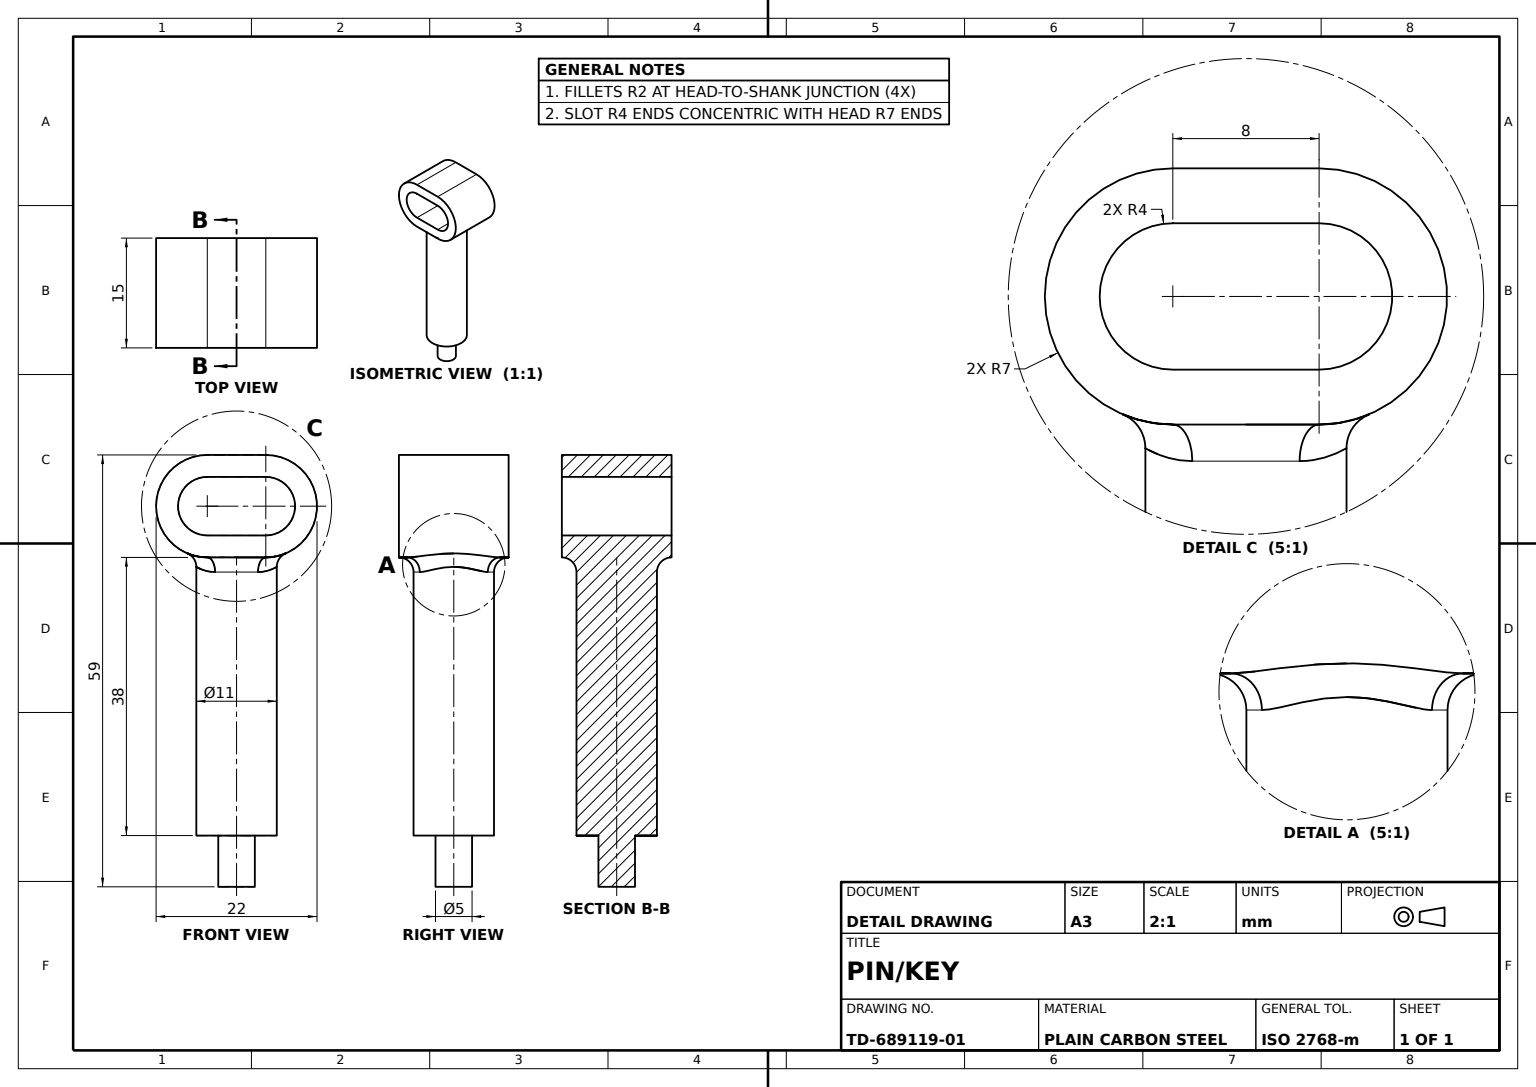
ISO-10303-21;
HEADER;
FILE_DESCRIPTION((''),'2;1');
FILE_NAME('','',(''),(''),'','','');
FILE_SCHEMA(('AUTOMOTIVE_DESIGN'));
ENDSEC;
DATA;
#1=APPLICATION_CONTEXT('');
#2=PRODUCT_CONTEXT('',#1,'mechanical');
#3=PRODUCT('','','',(#2));
#4=PRODUCT_DEFINITION_FORMATION('','',#3);
#5=PRODUCT_DEFINITION_CONTEXT('',#1,'design');
#6=PRODUCT_DEFINITION('','',#4,#5);
#7=PRODUCT_DEFINITION_SHAPE('','',#6);
#8=(LENGTH_UNIT()NAMED_UNIT(*)SI_UNIT(.MILLI.,.METRE.));
#9=(NAMED_UNIT(*)PLANE_ANGLE_UNIT()SI_UNIT($,.RADIAN.));
#10=(NAMED_UNIT(*)SI_UNIT($,.STERADIAN.)SOLID_ANGLE_UNIT());
#11=UNCERTAINTY_MEASURE_WITH_UNIT(LENGTH_MEASURE(1.E-05),#8,'distance_accuracy_value','');
#12=(GEOMETRIC_REPRESENTATION_CONTEXT(3)GLOBAL_UNCERTAINTY_ASSIGNED_CONTEXT((#11))GLOBAL_UNIT_ASSIGNED_CONTEXT((#8,#9,#10))REPRESENTATION_CONTEXT('',''));
#13=CARTESIAN_POINT('',(4.,-7.,-6.344289));
#14=VERTEX_POINT('',#13);
#15=CARTESIAN_POINT('',(4.,-7.,-7.5));
#16=VERTEX_POINT('',#15);
#17=CARTESIAN_POINT('',(4.,-7.,7.5));
#18=DIRECTION('',(0.,0.,-1.));
#19=VECTOR('',#18,1000.);
#20=LINE('',#17,#19);
#21=EDGE_CURVE('',#14,#16,#20,.T.);
#22=ORIENTED_EDGE('',*,*,#21,.F.);
#23=CARTESIAN_POINT('',(0.,-7.,-7.5));
#24=VERTEX_POINT('',#23);
#25=CARTESIAN_POINT('',(0.,-7.,0.));
#26=DIRECTION('',(0.,1.,0.));
#27=DIRECTION('',(-1.,0.,0.));
#28=AXIS2_PLACEMENT_3D('',#25,#26,#27);
#29=CIRCLE('',#28,7.5);
#30=EDGE_CURVE('',#14,#24,#29,.T.);
#31=ORIENTED_EDGE('',*,*,#30,.T.);
#32=CARTESIAN_POINT('',(-4.,-7.,-7.5));
#33=DIRECTION('',(1.,0.,0.));
#34=VECTOR('',#33,1000.);
#35=LINE('',#32,#34);
#36=EDGE_CURVE('',#24,#16,#35,.T.);
#37=ORIENTED_EDGE('',*,*,#36,.T.);
#38=EDGE_LOOP('',(#22,#31,#37));
#39=FACE_OUTER_BOUND('',#38,.T.);
#40=CARTESIAN_POINT('',(-4.,-7.,7.5));
#41=AXIS2_PLACEMENT_3D('',#40,#26,#27);
#42=PLANE('',#41);
#43=ADVANCED_FACE('',(#39),#42,.F.);
#44=CARTESIAN_POINT('',(4.,4.,7.5));
#45=VERTEX_POINT('',#44);
#46=CARTESIAN_POINT('',(-4.,4.,7.5));
#47=VERTEX_POINT('',#46);
#48=VECTOR('',#27,1000.);
#49=LINE('',#46,#48);
#50=EDGE_CURVE('',#45,#47,#49,.T.);
#51=ORIENTED_EDGE('',*,*,#50,.F.);
#52=CARTESIAN_POINT('',(4.,-4.,7.5));
#53=VERTEX_POINT('',#52);
#54=CARTESIAN_POINT('',(4.,0.,7.5));
#55=DIRECTION('',(0.,0.,1.));
#56=AXIS2_PLACEMENT_3D('',#54,#55,#33);
#57=CIRCLE('',#56,4.);
#58=EDGE_CURVE('',#53,#45,#57,.T.);
#59=ORIENTED_EDGE('',*,*,#58,.F.);
#60=CARTESIAN_POINT('',(-4.,-4.,7.5));
#61=VERTEX_POINT('',#60);
#62=LINE('',#60,#34);
#63=EDGE_CURVE('',#61,#53,#62,.T.);
#64=ORIENTED_EDGE('',*,*,#63,.F.);
#65=CARTESIAN_POINT('',(-8.,0.,7.5));
#66=VERTEX_POINT('',#65);
#67=CARTESIAN_POINT('',(-4.,0.,7.5));
#68=AXIS2_PLACEMENT_3D('',#67,#55,#33);
#69=CIRCLE('',#68,4.);
#70=EDGE_CURVE('',#66,#61,#69,.T.);
#71=ORIENTED_EDGE('',*,*,#70,.F.);
#72=EDGE_CURVE('',#47,#66,#69,.T.);
#73=ORIENTED_EDGE('',*,*,#72,.F.);
#74=EDGE_LOOP('',(#51,#59,#64,#71,#73));
#75=FACE_BOUND('',#74,.T.);
#76=VERTEX_POINT('',#40);
#77=CARTESIAN_POINT('',(0.,-7.,7.5));
#78=VERTEX_POINT('',#77);
#79=LINE('',#40,#34);
#80=EDGE_CURVE('',#76,#78,#79,.T.);
#81=ORIENTED_EDGE('',*,*,#80,.T.);
#82=VERTEX_POINT('',#17);
#83=EDGE_CURVE('',#78,#82,#79,.T.);
#84=ORIENTED_EDGE('',*,*,#83,.T.);
#85=CARTESIAN_POINT('',(4.,7.,7.5));
#86=VERTEX_POINT('',#85);
#87=CIRCLE('',#56,7.);
#88=EDGE_CURVE('',#82,#86,#87,.T.);
#89=ORIENTED_EDGE('',*,*,#88,.T.);
#90=CARTESIAN_POINT('',(-4.,7.,7.5));
#91=VERTEX_POINT('',#90);
#92=LINE('',#90,#48);
#93=EDGE_CURVE('',#86,#91,#92,.T.);
#94=ORIENTED_EDGE('',*,*,#93,.T.);
#95=CARTESIAN_POINT('',(-11.,0.,7.5));
#96=VERTEX_POINT('',#95);
#97=CIRCLE('',#68,7.);
#98=EDGE_CURVE('',#91,#96,#97,.T.);
#99=ORIENTED_EDGE('',*,*,#98,.T.);
#100=EDGE_CURVE('',#96,#76,#97,.T.);
#101=ORIENTED_EDGE('',*,*,#100,.T.);
#102=EDGE_LOOP('',(#81,#84,#89,#94,#99,#101));
#103=FACE_OUTER_BOUND('',#102,.T.);
#104=PLANE('',#68);
#105=ADVANCED_FACE('',(#75,#103),#104,.T.);
#106=ORIENTED_EDGE('',*,*,#63,.T.);
#107=CARTESIAN_POINT('',(4.,-4.,-7.5));
#108=VERTEX_POINT('',#107);
#109=LINE('',#52,#19);
#110=EDGE_CURVE('',#53,#108,#109,.T.);
#111=ORIENTED_EDGE('',*,*,#110,.T.);
#112=CARTESIAN_POINT('',(-4.,-4.,-7.5));
#113=VERTEX_POINT('',#112);
#114=LINE('',#112,#34);
#115=EDGE_CURVE('',#113,#108,#114,.T.);
#116=ORIENTED_EDGE('',*,*,#115,.F.);
#117=LINE('',#60,#19);
#118=EDGE_CURVE('',#61,#113,#117,.T.);
#119=ORIENTED_EDGE('',*,*,#118,.F.);
#120=EDGE_LOOP('',(#106,#111,#116,#119));
#121=FACE_OUTER_BOUND('',#120,.T.);
#122=AXIS2_PLACEMENT_3D('',#60,#26,#27);
#123=PLANE('',#122);
#124=ADVANCED_FACE('',(#121),#123,.T.);
#125=CARTESIAN_POINT('',(-2.933333,-9.,4.652478));
#126=VERTEX_POINT('',#125);
#127=CARTESIAN_POINT('',(-4.,-7.,6.344289));
#128=VERTEX_POINT('',#127);
#129=CARTESIAN_POINT('',(-4.,-9.,6.344289));
#130=DIRECTION('',(0.845905169,0.,0.533333333));
#131=DIRECTION('',(0.533333333,0.,-0.845905169));
#132=AXIS2_PLACEMENT_3D('',#129,#130,#131);
#133=CIRCLE('',#132,2.);
#134=EDGE_CURVE('',#126,#128,#133,.T.);
#135=ORIENTED_EDGE('',*,*,#134,.F.);
#136=CARTESIAN_POINT('',(2.933333,-9.,4.652478));
#137=VERTEX_POINT('',#136);
#138=CARTESIAN_POINT('',(0.,-9.,0.));
#139=DIRECTION('',(0.,-1.,0.));
#140=AXIS2_PLACEMENT_3D('',#138,#139,#27);
#141=CIRCLE('',#140,5.5);
#142=EDGE_CURVE('',#137,#126,#141,.T.);
#143=ORIENTED_EDGE('',*,*,#142,.F.);
#144=CARTESIAN_POINT('',(4.,-7.,6.344289));
#145=VERTEX_POINT('',#144);
#146=CARTESIAN_POINT('',(4.,-9.,6.344289));
#147=DIRECTION('',(-0.845905169,0.,0.533333333));
#148=DIRECTION('',(0.533333333,0.,0.845905169));
#149=AXIS2_PLACEMENT_3D('',#146,#147,#148);
#150=CIRCLE('',#149,2.);
#151=EDGE_CURVE('',#145,#137,#150,.T.);
#152=ORIENTED_EDGE('',*,*,#151,.F.);
#153=EDGE_CURVE('',#78,#145,#29,.T.);
#154=ORIENTED_EDGE('',*,*,#153,.F.);
#155=EDGE_CURVE('',#128,#78,#29,.T.);
#156=ORIENTED_EDGE('',*,*,#155,.F.);
#157=EDGE_LOOP('',(#135,#143,#152,#154,#156));
#158=FACE_OUTER_BOUND('',#157,.T.);
#159=AXIS2_PLACEMENT_3D('',#138,#26,#27);
#160=TOROIDAL_SURFACE('',#159,7.5,2.);
#161=ADVANCED_FACE('',(#158),#160,.F.);
#162=ORIENTED_EDGE('',*,*,#83,.F.);
#163=ORIENTED_EDGE('',*,*,#153,.T.);
#164=EDGE_CURVE('',#82,#145,#20,.T.);
#165=ORIENTED_EDGE('',*,*,#164,.F.);
#166=EDGE_LOOP('',(#162,#163,#165));
#167=FACE_OUTER_BOUND('',#166,.T.);
#168=ADVANCED_FACE('',(#167),#42,.F.);
#169=CARTESIAN_POINT('',(2.933333,-9.,-4.652478));
#170=VERTEX_POINT('',#169);
#171=CARTESIAN_POINT('',(5.5,-8.291562,0.));
#172=VERTEX_POINT('',#171);
#173=CARTESIAN_POINT('',(3.133043,-9.,-4.526564));
#174=CARTESIAN_POINT('',(3.324343,-8.987525,-4.387772));
#175=CARTESIAN_POINT('',(3.681966,-8.945264,-4.092301));
#176=CARTESIAN_POINT('',(3.84954,-8.915501,-3.934916));
#177=CARTESIAN_POINT('',(4.320562,-8.809648,-3.43407));
#178=CARTESIAN_POINT('',(4.59485,-8.715803,-3.05715));
#179=CARTESIAN_POINT('',(4.925989,-8.581444,-2.456998));
#180=CARTESIAN_POINT('',(5.023745,-8.53753,-2.25051));
#181=CARTESIAN_POINT('',(5.193968,-8.456487,-1.823596));
#182=CARTESIAN_POINT('',(5.266775,-8.419162,-1.601479));
#183=CARTESIAN_POINT('',(5.440779,-8.326918,-0.928725));
#184=CARTESIAN_POINT('',(5.5,-8.291562,-0.470006));
#185=B_SPLINE_CURVE_WITH_KNOTS('',3,(#169,#173,#174,#175,#176,#177,#178,#179,#180,#181,#182,#183,#184,#171),.UNSPECIFIED.,.F.,.F.,(4,2,2,2,2,2,4),(0.,0.000707891,0.001415783,0.002831566,0.003539457,0.004247348,0.005663131),.UNSPECIFIED.);
#186=EDGE_CURVE('',#170,#172,#185,.T.);
#187=ORIENTED_EDGE('',*,*,#186,.F.);
#188=CARTESIAN_POINT('',(4.,-9.,-6.344289));
#189=AXIS2_PLACEMENT_3D('',#188,#130,#131);
#190=CIRCLE('',#189,2.);
#191=EDGE_CURVE('',#14,#170,#190,.T.);
#192=ORIENTED_EDGE('',*,*,#191,.F.);
#193=CARTESIAN_POINT('',(4.468237,-7.,5.964722));
#194=CARTESIAN_POINT('',(4.865103,-6.955024,5.526591));
#195=CARTESIAN_POINT('',(5.378548,-6.865114,4.799618));
#196=CARTESIAN_POINT('',(5.535888,-6.830968,4.544603));
#197=CARTESIAN_POINT('',(5.817747,-6.761425,4.023897));
#198=CARTESIAN_POINT('',(5.943356,-6.725845,3.756806));
#199=CARTESIAN_POINT('',(6.278059,-6.623061,2.936233));
#200=CARTESIAN_POINT('',(6.445689,-6.55993,2.359248));
#201=CARTESIAN_POINT('',(6.666602,-6.473277,1.194519));
#202=CARTESIAN_POINT('',(6.722103,-6.449043,0.600743));
#203=CARTESIAN_POINT('',(6.722341,-6.448942,-0.596899));
#204=CARTESIAN_POINT('',(6.667486,-6.472915,-1.188495));
#205=CARTESIAN_POINT('',(6.501583,-6.538013,-2.065229));
#206=CARTESIAN_POINT('',(6.431801,-6.564616,-2.356752));
#207=CARTESIAN_POINT('',(6.264949,-6.624036,-2.92676));
#208=CARTESIAN_POINT('',(6.167832,-6.656884,-3.206115));
#209=CARTESIAN_POINT('',(5.833401,-6.759663,-4.027076));
#210=CARTESIAN_POINT('',(5.549791,-6.835022,-4.556645));
#211=CARTESIAN_POINT('',(5.039313,-6.92457,-5.280187));
#212=CARTESIAN_POINT('',(4.854699,-6.950556,-5.510504));
#213=CARTESIAN_POINT('',(4.452763,-6.988258,-5.947148));
#214=CARTESIAN_POINT('',(4.234007,-7.,-6.154596));
#215=B_SPLINE_CURVE_WITH_KNOTS('',3,(#144,#193,#194,#195,#196,#197,#198,#199,#200,#201,#202,#203,#204,#205,#206,#207,#208,#209,#210,#211,#212,#213,#214,#13),.UNSPECIFIED.,.F.,.F.,(4,2,2,2,2,2,2,2,2,2,2,4),(0.,0.001778288,0.002667432,0.003556577,0.005334865,0.007113153,0.008891442,0.009780586,0.01066973,0.012448018,0.013337162,0.014226307),.UNSPECIFIED.);
#216=EDGE_CURVE('',#145,#14,#215,.T.);
#217=ORIENTED_EDGE('',*,*,#216,.F.);
#218=ORIENTED_EDGE('',*,*,#151,.T.);
#219=CARTESIAN_POINT('',(5.5,-8.291562,0.23522));
#220=CARTESIAN_POINT('',(5.484785,-8.300403,0.469857));
#221=CARTESIAN_POINT('',(5.425872,-8.333622,0.929272));
#222=CARTESIAN_POINT('',(5.382182,-8.357987,1.15548));
#223=CARTESIAN_POINT('',(5.266772,-8.419159,1.601289));
#224=CARTESIAN_POINT('',(5.194588,-8.456191,1.822026));
#225=CARTESIAN_POINT('',(5.023221,-8.53778,2.251839));
#226=CARTESIAN_POINT('',(4.925051,-8.581848,2.458861));
#227=CARTESIAN_POINT('',(4.704312,-8.671365,2.858598));
#228=CARTESIAN_POINT('',(4.581742,-8.716834,3.051308));
#229=CARTESIAN_POINT('',(4.311141,-8.803745,3.422997));
#230=CARTESIAN_POINT('',(4.162384,-8.845267,3.602452));
#231=CARTESIAN_POINT('',(3.688497,-8.951547,4.105776));
#232=CARTESIAN_POINT('',(3.333153,-9.,4.400396));
#233=B_SPLINE_CURVE_WITH_KNOTS('',3,(#171,#219,#220,#221,#222,#223,#224,#225,#226,#227,#228,#229,#230,#231,#232,#136),.UNSPECIFIED.,.F.,.F.,(4,2,2,2,2,2,2,4),(0.005663131,0.006371677,0.007080223,0.007788769,0.008497314,0.00920586,0.009914406,0.011331498),.UNSPECIFIED.);
#234=EDGE_CURVE('',#172,#137,#233,.T.);
#235=ORIENTED_EDGE('',*,*,#234,.F.);
#236=EDGE_LOOP('',(#187,#192,#217,#218,#235));
#237=FACE_OUTER_BOUND('',#236,.T.);
#238=CARTESIAN_POINT('',(2.933333,-7.,4.652478));
#239=CARTESIAN_POINT('',(4.421288,-7.,6.002781));
#240=CARTESIAN_POINT('',(3.238913,-7.06306,4.459814));
#241=CARTESIAN_POINT('',(3.330464,-9.,4.402092));
#242=CARTESIAN_POINT('',(4.79799,-6.962674,5.602232));
#243=CARTESIAN_POINT('',(3.553947,-7.102304,4.223306));
#244=CARTESIAN_POINT('',(3.685723,-8.952009,4.108303));
#245=CARTESIAN_POINT('',(5.301296,-6.880082,4.915778));
#246=CARTESIAN_POINT('',(4.017096,-7.122128,3.768812));
#247=CARTESIAN_POINT('',(4.16027,-8.84582,3.604904));
#248=CARTESIAN_POINT('',(5.459491,-6.847756,4.670729));
#249=CARTESIAN_POINT('',(4.168117,-7.122554,3.602781));
#250=CARTESIAN_POINT('',(4.309425,-8.804258,3.425202));
#251=CARTESIAN_POINT('',(5.747471,-6.779987,4.162566));
#252=CARTESIAN_POINT('',(4.451479,-7.113522,3.246293));
#253=CARTESIAN_POINT('',(4.580949,-8.717126,3.052549));
#254=CARTESIAN_POINT('',(5.87798,-6.744494,3.898869));
#255=CARTESIAN_POINT('',(4.584829,-7.104349,3.055827));
#256=CARTESIAN_POINT('',(4.704001,-8.671493,2.85917));
#257=CARTESIAN_POINT('',(6.112868,-6.674639,3.351956));
#258=CARTESIAN_POINT('',(4.829413,-7.080665,2.6509));
#259=CARTESIAN_POINT('',(4.925466,-8.581678,2.458101));
#260=CARTESIAN_POINT('',(6.217247,-6.640264,3.068744));
#261=CARTESIAN_POINT('',(4.941295,-7.066219,2.436349));
#262=CARTESIAN_POINT('',(5.02388,-8.537482,2.250412));
#263=CARTESIAN_POINT('',(6.399176,-6.576719,2.481446));
#264=CARTESIAN_POINT('',(5.138466,-7.03651,1.983848));
#265=CARTESIAN_POINT('',(5.195414,-8.455782,1.819727));
#266=CARTESIAN_POINT('',(6.475653,-6.547934,2.180199));
#267=CARTESIAN_POINT('',(5.223258,-7.021409,1.747557));
#268=CARTESIAN_POINT('',(5.26752,-8.418772,1.598813));
#269=CARTESIAN_POINT('',(6.597792,-6.500444,1.572459));
#270=CARTESIAN_POINT('',(5.359166,-6.995401,1.26649));
#271=CARTESIAN_POINT('',(5.38268,-8.357713,1.153137));
#272=CARTESIAN_POINT('',(6.643932,-6.481571,1.264462));
#273=CARTESIAN_POINT('',(5.411371,-6.984344,1.019681));
#274=CARTESIAN_POINT('',(5.426183,-8.333448,0.927272));
#275=CARTESIAN_POINT('',(6.706105,-6.45586,0.639935));
#276=CARTESIAN_POINT('',(5.481585,-6.969134,0.517636));
#277=CARTESIAN_POINT('',(5.484803,-8.300392,0.469286));
#278=CARTESIAN_POINT('',(6.722131,-6.449031,0.32171));
#279=CARTESIAN_POINT('',(5.499897,-6.964935,0.259943));
#280=CARTESIAN_POINT('',(5.499914,-8.291611,0.23592));
#281=CARTESIAN_POINT('',(6.722403,-6.448916,-0.635218));
#282=CARTESIAN_POINT('',(5.500205,-6.964866,-0.513249));
#283=CARTESIAN_POINT('',(5.50017,-8.291464,-0.465826));
#284=CARTESIAN_POINT('',(6.660312,-6.476113,-1.259635));
#285=CARTESIAN_POINT('',(5.427824,-6.982239,-1.022098));
#286=CARTESIAN_POINT('',(5.441627,-8.326431,-0.923732));
#287=CARTESIAN_POINT('',(6.476428,-6.547643,-2.177202));
#288=CARTESIAN_POINT('',(5.22411,-7.021258,-1.745223));
#289=CARTESIAN_POINT('',(5.268251,-8.418398,-1.596615));
#290=CARTESIAN_POINT('',(6.399361,-6.576642,-2.48053));
#291=CARTESIAN_POINT('',(5.138684,-7.036463,-1.983102));
#292=CARTESIAN_POINT('',(5.195588,-8.455683,-1.819055));
#293=CARTESIAN_POINT('',(6.218679,-6.639776,-3.064436));
#294=CARTESIAN_POINT('',(4.942847,-7.066,-2.433034));
#295=CARTESIAN_POINT('',(5.025231,-8.536854,-2.247253));
#296=CARTESIAN_POINT('',(6.114734,-6.674049,-3.347191));
#297=CARTESIAN_POINT('',(4.831385,-7.080436,-2.647328));
#298=CARTESIAN_POINT('',(4.927225,-8.58092,-2.454607));
#299=CARTESIAN_POINT('',(5.879749,-6.744003,-3.895164));
#300=CARTESIAN_POINT('',(4.58664,-7.104212,-3.053137));
#301=CARTESIAN_POINT('',(4.705668,-8.67086,-2.856454));
#302=CARTESIAN_POINT('',(5.748195,-6.779817,-4.161288));
#303=CARTESIAN_POINT('',(4.452178,-7.113499,-3.245412));
#304=CARTESIAN_POINT('',(4.581632,-8.716907,-3.051611));
#305=CARTESIAN_POINT('',(5.458785,-6.847923,-4.671976));
#306=CARTESIAN_POINT('',(4.167409,-7.122577,-3.603673));
#307=CARTESIAN_POINT('',(4.30876,-8.804472,-3.426116));
#308=CARTESIAN_POINT('',(5.302904,-6.879756,-4.913299));
#309=CARTESIAN_POINT('',(4.018641,-7.122135,-3.76712));
#310=CARTESIAN_POINT('',(4.161786,-8.845401,-3.603086));
#311=CARTESIAN_POINT('',(4.802236,-6.9621,-5.597005));
#312=CARTESIAN_POINT('',(3.557744,-7.102586,-4.219937));
#313=CARTESIAN_POINT('',(3.689728,-8.951272,-4.10447));
#314=CARTESIAN_POINT('',(4.42382,-7.,-6.000728));
#315=CARTESIAN_POINT('',(3.240693,-7.063428,-4.458692));
#316=CARTESIAN_POINT('',(3.332876,-9.,-4.400572));
#317=CARTESIAN_POINT('',(2.933333,-7.,-4.652478));
#318=(BOUNDED_SURFACE()B_SPLINE_SURFACE(3,2,((#144,#238,#136),(#239,#240,#241),(#242,#243,#244),(#245,#246,#247),(#248,#249,#250),(#251,#252,#253),(#254,#255,#256),(#257,#258,#259),(#260,#261,#262),(#263,#264,#265),(#266,#267,#268),(#269,#270,#271),(#272,#273,#274),(#275,#276,#277),(#278,#279,#280),(#281,#282,#283),(#284,#285,#286),(#287,#288,#289),(#290,#291,#292),(#293,#294,#295),(#296,#297,#298),(#299,#300,#301),(#302,#303,#304),(#305,#306,#307),(#308,#309,#310),(#311,#312,#313),(#314,#315,#316),(#13,#317,#169)),.UNSPECIFIED.,.F.,.F.,.F.)B_SPLINE_SURFACE_WITH_KNOTS((4,2,2,2,2,2,2,2,2,2,2,2,2,4),(3,3),(0.,0.001889948,0.002834922,0.003779896,0.004724871,0.005669845,0.006614819,0.007559793,0.009449741,0.010394715,0.011339689,0.012284663,0.013229637,0.015119586),(0.,1.),.UNSPECIFIED.)GEOMETRIC_REPRESENTATION_ITEM()RATIONAL_B_SPLINE_SURFACE(((1.,0.707106781,1.),(1.,0.718485878,1.),(1.,0.732827948,1.),(1.,0.754995566,1.),(1.,0.762549128,1.),(1.,0.777020285,1.),(1.,0.783964533,1.),(1.,0.796885728,1.),(1.,0.80286471,1.),(1.,0.813514846,1.),(1.,0.818123471,1.),(1.,0.825570539,1.),(1.,0.828438021,1.),(1.,0.83231667,1.),(1.,0.833327624,1.),(1.,0.833344678,1.),(1.,0.829383755,1.),(1.,0.818170092,1.),(1.,0.813526465,1.),(1.,0.802947783,1.),(1.,0.79699087,1.),(1.,0.784059367,1.),(1.,0.777056669,1.),(1.,0.762513647,1.),(1.,0.755072161,1.),(1.,0.733003591,1.),(1.,0.718556253,1.),(1.,0.707106781,1.)))REPRESENTATION_ITEM('')SURFACE());
#319=ADVANCED_FACE('',(#237),#318,.F.);
#320=CARTESIAN_POINT('',(4.,4.,-7.5));
#321=VERTEX_POINT('',#320);
#322=CARTESIAN_POINT('',(-4.,4.,-7.5));
#323=VERTEX_POINT('',#322);
#324=LINE('',#322,#48);
#325=EDGE_CURVE('',#321,#323,#324,.T.);
#326=ORIENTED_EDGE('',*,*,#325,.F.);
#327=LINE('',#44,#19);
#328=EDGE_CURVE('',#45,#321,#327,.T.);
#329=ORIENTED_EDGE('',*,*,#328,.F.);
#330=ORIENTED_EDGE('',*,*,#50,.T.);
#331=LINE('',#46,#19);
#332=EDGE_CURVE('',#47,#323,#331,.T.);
#333=ORIENTED_EDGE('',*,*,#332,.T.);
#334=EDGE_LOOP('',(#326,#329,#330,#333));
#335=FACE_OUTER_BOUND('',#334,.T.);
#336=AXIS2_PLACEMENT_3D('',#46,#139,#18);
#337=PLANE('',#336);
#338=ADVANCED_FACE('',(#335),#337,.T.);
#339=CARTESIAN_POINT('',(4.,7.,-7.5));
#340=VERTEX_POINT('',#339);
#341=LINE('',#85,#19);
#342=EDGE_CURVE('',#86,#340,#341,.T.);
#343=ORIENTED_EDGE('',*,*,#342,.T.);
#344=CARTESIAN_POINT('',(-4.,7.,-7.5));
#345=VERTEX_POINT('',#344);
#346=LINE('',#344,#48);
#347=EDGE_CURVE('',#340,#345,#346,.T.);
#348=ORIENTED_EDGE('',*,*,#347,.T.);
#349=LINE('',#90,#19);
#350=EDGE_CURVE('',#91,#345,#349,.T.);
#351=ORIENTED_EDGE('',*,*,#350,.F.);
#352=ORIENTED_EDGE('',*,*,#93,.F.);
#353=EDGE_LOOP('',(#343,#348,#351,#352));
#354=FACE_OUTER_BOUND('',#353,.T.);
#355=AXIS2_PLACEMENT_3D('',#90,#139,#18);
#356=PLANE('',#355);
#357=ADVANCED_FACE('',(#354),#356,.F.);
#358=CARTESIAN_POINT('',(-2.933333,-9.,-4.652478));
#359=VERTEX_POINT('',#358);
#360=EDGE_CURVE('',#359,#170,#141,.T.);
#361=ORIENTED_EDGE('',*,*,#360,.T.);
#362=ORIENTED_EDGE('',*,*,#186,.T.);
#363=CARTESIAN_POINT('',(5.5,-45.,0.));
#364=VERTEX_POINT('',#363);
#365=VECTOR('',#26,1000.);
#366=LINE('',#363,#365);
#367=EDGE_CURVE('',#364,#172,#366,.T.);
#368=ORIENTED_EDGE('',*,*,#367,.F.);
#369=CARTESIAN_POINT('',(-5.5,-45.,0.));
#370=VERTEX_POINT('',#369);
#371=CARTESIAN_POINT('',(0.,-45.,0.));
#372=AXIS2_PLACEMENT_3D('',#371,#139,#33);
#373=CIRCLE('',#372,5.5);
#374=EDGE_CURVE('',#370,#364,#373,.T.);
#375=ORIENTED_EDGE('',*,*,#374,.F.);
#376=CARTESIAN_POINT('',(-5.5,-8.291562,0.));
#377=VERTEX_POINT('',#376);
#378=LINE('',#369,#365);
#379=EDGE_CURVE('',#370,#377,#378,.T.);
#380=ORIENTED_EDGE('',*,*,#379,.T.);
#381=CARTESIAN_POINT('',(-5.5,-8.291562,-0.23522));
#382=CARTESIAN_POINT('',(-5.484785,-8.300403,-0.469857));
#383=CARTESIAN_POINT('',(-5.425872,-8.333622,-0.929272));
#384=CARTESIAN_POINT('',(-5.382182,-8.357987,-1.15548));
#385=CARTESIAN_POINT('',(-5.266772,-8.419159,-1.601289));
#386=CARTESIAN_POINT('',(-5.194588,-8.456191,-1.822026));
#387=CARTESIAN_POINT('',(-5.023221,-8.53778,-2.251839));
#388=CARTESIAN_POINT('',(-4.925051,-8.581848,-2.458861));
#389=CARTESIAN_POINT('',(-4.704312,-8.671365,-2.858598));
#390=CARTESIAN_POINT('',(-4.581742,-8.716834,-3.051308));
#391=CARTESIAN_POINT('',(-4.311141,-8.803745,-3.422997));
#392=CARTESIAN_POINT('',(-4.162384,-8.845267,-3.602452));
#393=CARTESIAN_POINT('',(-3.688497,-8.951547,-4.105776));
#394=CARTESIAN_POINT('',(-3.333153,-9.,-4.400396));
#395=B_SPLINE_CURVE_WITH_KNOTS('',3,(#376,#381,#382,#383,#384,#385,#386,#387,#388,#389,#390,#391,#392,#393,#394,#358),.UNSPECIFIED.,.F.,.F.,(4,2,2,2,2,2,2,4),(0.005663131,0.006371677,0.007080223,0.007788769,0.008497314,0.00920586,0.009914406,0.011331498),.UNSPECIFIED.);
#396=EDGE_CURVE('',#377,#359,#395,.T.);
#397=ORIENTED_EDGE('',*,*,#396,.T.);
#398=EDGE_LOOP('',(#361,#362,#368,#375,#380,#397));
#399=FACE_OUTER_BOUND('',#398,.T.);
#400=AXIS2_PLACEMENT_3D('',#371,#26,#27);
#401=CYLINDRICAL_SURFACE('',#400,5.5);
#402=ADVANCED_FACE('',(#399),#401,.T.);
#403=ORIENTED_EDGE('',*,*,#115,.T.);
#404=CARTESIAN_POINT('',(4.,0.,-7.5));
#405=AXIS2_PLACEMENT_3D('',#404,#55,#33);
#406=CIRCLE('',#405,4.);
#407=EDGE_CURVE('',#108,#321,#406,.T.);
#408=ORIENTED_EDGE('',*,*,#407,.T.);
#409=ORIENTED_EDGE('',*,*,#325,.T.);
#410=CARTESIAN_POINT('',(-8.,0.,-7.5));
#411=VERTEX_POINT('',#410);
#412=CARTESIAN_POINT('',(-4.,0.,-7.5));
#413=AXIS2_PLACEMENT_3D('',#412,#55,#33);
#414=CIRCLE('',#413,4.);
#415=EDGE_CURVE('',#323,#411,#414,.T.);
#416=ORIENTED_EDGE('',*,*,#415,.T.);
#417=EDGE_CURVE('',#411,#113,#414,.T.);
#418=ORIENTED_EDGE('',*,*,#417,.T.);
#419=EDGE_LOOP('',(#403,#408,#409,#416,#418));
#420=FACE_BOUND('',#419,.T.);
#421=CARTESIAN_POINT('',(-11.,0.,-7.5));
#422=VERTEX_POINT('',#421);
#423=VERTEX_POINT('',#32);
#424=CIRCLE('',#413,7.);
#425=EDGE_CURVE('',#422,#423,#424,.T.);
#426=ORIENTED_EDGE('',*,*,#425,.F.);
#427=EDGE_CURVE('',#345,#422,#424,.T.);
#428=ORIENTED_EDGE('',*,*,#427,.F.);
#429=ORIENTED_EDGE('',*,*,#347,.F.);
#430=CIRCLE('',#405,7.);
#431=EDGE_CURVE('',#16,#340,#430,.T.);
#432=ORIENTED_EDGE('',*,*,#431,.F.);
#433=ORIENTED_EDGE('',*,*,#36,.F.);
#434=EDGE_CURVE('',#423,#24,#35,.T.);
#435=ORIENTED_EDGE('',*,*,#434,.F.);
#436=EDGE_LOOP('',(#426,#428,#429,#432,#433,#435));
#437=FACE_OUTER_BOUND('',#436,.T.);
#438=PLANE('',#413);
#439=ADVANCED_FACE('',(#420,#437),#438,.F.);
#440=ORIENTED_EDGE('',*,*,#434,.T.);
#441=CARTESIAN_POINT('',(-4.,-7.,-6.344289));
#442=VERTEX_POINT('',#441);
#443=EDGE_CURVE('',#24,#442,#29,.T.);
#444=ORIENTED_EDGE('',*,*,#443,.T.);
#445=LINE('',#40,#19);
#446=EDGE_CURVE('',#442,#423,#445,.T.);
#447=ORIENTED_EDGE('',*,*,#446,.T.);
#448=EDGE_LOOP('',(#440,#444,#447));
#449=FACE_OUTER_BOUND('',#448,.T.);
#450=ADVANCED_FACE('',(#449),#42,.F.);
#451=CARTESIAN_POINT('',(-3.133043,-9.,4.526564));
#452=CARTESIAN_POINT('',(-3.324343,-8.987525,4.387772));
#453=CARTESIAN_POINT('',(-3.681966,-8.945264,4.092301));
#454=CARTESIAN_POINT('',(-3.84954,-8.915501,3.934916));
#455=CARTESIAN_POINT('',(-4.320562,-8.809648,3.43407));
#456=CARTESIAN_POINT('',(-4.59485,-8.715803,3.05715));
#457=CARTESIAN_POINT('',(-4.925989,-8.581444,2.456998));
#458=CARTESIAN_POINT('',(-5.023745,-8.53753,2.25051));
#459=CARTESIAN_POINT('',(-5.193968,-8.456487,1.823596));
#460=CARTESIAN_POINT('',(-5.266775,-8.419162,1.601479));
#461=CARTESIAN_POINT('',(-5.440779,-8.326918,0.928725));
#462=CARTESIAN_POINT('',(-5.5,-8.291562,0.470006));
#463=B_SPLINE_CURVE_WITH_KNOTS('',3,(#125,#451,#452,#453,#454,#455,#456,#457,#458,#459,#460,#461,#462,#376),.UNSPECIFIED.,.F.,.F.,(4,2,2,2,2,2,4),(0.,0.000707891,0.001415783,0.002831566,0.003539457,0.004247348,0.005663131),.UNSPECIFIED.);
#464=EDGE_CURVE('',#126,#377,#463,.T.);
#465=ORIENTED_EDGE('',*,*,#464,.T.);
#466=ORIENTED_EDGE('',*,*,#379,.F.);
#467=EDGE_CURVE('',#364,#370,#373,.T.);
#468=ORIENTED_EDGE('',*,*,#467,.F.);
#469=ORIENTED_EDGE('',*,*,#367,.T.);
#470=ORIENTED_EDGE('',*,*,#234,.T.);
#471=ORIENTED_EDGE('',*,*,#142,.T.);
#472=EDGE_LOOP('',(#465,#466,#468,#469,#470,#471));
#473=FACE_OUTER_BOUND('',#472,.T.);
#474=ADVANCED_FACE('',(#473),#401,.T.);
#475=CARTESIAN_POINT('',(-2.5,-52.,0.));
#476=VERTEX_POINT('',#475);
#477=CARTESIAN_POINT('',(-2.5,-45.,0.));
#478=VERTEX_POINT('',#477);
#479=LINE('',#475,#365);
#480=EDGE_CURVE('',#476,#478,#479,.T.);
#481=ORIENTED_EDGE('',*,*,#480,.F.);
#482=CARTESIAN_POINT('',(2.5,-52.,0.));
#483=VERTEX_POINT('',#482);
#484=CARTESIAN_POINT('',(0.,-52.,0.));
#485=AXIS2_PLACEMENT_3D('',#484,#139,#33);
#486=CIRCLE('',#485,2.5);
#487=EDGE_CURVE('',#483,#476,#486,.T.);
#488=ORIENTED_EDGE('',*,*,#487,.F.);
#489=CARTESIAN_POINT('',(2.5,-45.,0.));
#490=VERTEX_POINT('',#489);
#491=LINE('',#482,#365);
#492=EDGE_CURVE('',#483,#490,#491,.T.);
#493=ORIENTED_EDGE('',*,*,#492,.T.);
#494=CIRCLE('',#372,2.5);
#495=EDGE_CURVE('',#490,#478,#494,.T.);
#496=ORIENTED_EDGE('',*,*,#495,.T.);
#497=EDGE_LOOP('',(#481,#488,#493,#496));
#498=FACE_OUTER_BOUND('',#497,.T.);
#499=AXIS2_PLACEMENT_3D('',#484,#26,#27);
#500=CYLINDRICAL_SURFACE('',#499,2.5);
#501=ADVANCED_FACE('',(#498),#500,.T.);
#502=LINE('',#95,#19);
#503=EDGE_CURVE('',#96,#422,#502,.T.);
#504=ORIENTED_EDGE('',*,*,#503,.F.);
#505=ORIENTED_EDGE('',*,*,#98,.F.);
#506=ORIENTED_EDGE('',*,*,#350,.T.);
#507=ORIENTED_EDGE('',*,*,#427,.T.);
#508=EDGE_LOOP('',(#504,#505,#506,#507));
#509=FACE_OUTER_BOUND('',#508,.T.);
#510=AXIS2_PLACEMENT_3D('',#67,#18,#27);
#511=CYLINDRICAL_SURFACE('',#510,7.);
#512=ADVANCED_FACE('',(#509),#511,.T.);
#513=ORIENTED_EDGE('',*,*,#342,.F.);
#514=ORIENTED_EDGE('',*,*,#88,.F.);
#515=ORIENTED_EDGE('',*,*,#164,.T.);
#516=ORIENTED_EDGE('',*,*,#216,.T.);
#517=ORIENTED_EDGE('',*,*,#21,.T.);
#518=ORIENTED_EDGE('',*,*,#431,.T.);
#519=EDGE_LOOP('',(#513,#514,#515,#516,#517,#518));
#520=FACE_OUTER_BOUND('',#519,.T.);
#521=AXIS2_PLACEMENT_3D('',#54,#18,#27);
#522=CYLINDRICAL_SURFACE('',#521,7.);
#523=ADVANCED_FACE('',(#520),#522,.T.);
#524=ORIENTED_EDGE('',*,*,#425,.T.);
#525=ORIENTED_EDGE('',*,*,#446,.F.);
#526=CARTESIAN_POINT('',(-4.468237,-7.,-5.964722));
#527=CARTESIAN_POINT('',(-4.865103,-6.955024,-5.526591));
#528=CARTESIAN_POINT('',(-5.378548,-6.865114,-4.799618));
#529=CARTESIAN_POINT('',(-5.535888,-6.830968,-4.544603));
#530=CARTESIAN_POINT('',(-5.817747,-6.761425,-4.023897));
#531=CARTESIAN_POINT('',(-5.943356,-6.725845,-3.756806));
#532=CARTESIAN_POINT('',(-6.278059,-6.623061,-2.936233));
#533=CARTESIAN_POINT('',(-6.445689,-6.55993,-2.359248));
#534=CARTESIAN_POINT('',(-6.666602,-6.473277,-1.194519));
#535=CARTESIAN_POINT('',(-6.722103,-6.449043,-0.600743));
#536=CARTESIAN_POINT('',(-6.722341,-6.448942,0.596899));
#537=CARTESIAN_POINT('',(-6.667486,-6.472915,1.188495));
#538=CARTESIAN_POINT('',(-6.501583,-6.538013,2.065229));
#539=CARTESIAN_POINT('',(-6.431801,-6.564616,2.356752));
#540=CARTESIAN_POINT('',(-6.264949,-6.624036,2.92676));
#541=CARTESIAN_POINT('',(-6.167832,-6.656884,3.206115));
#542=CARTESIAN_POINT('',(-5.833401,-6.759663,4.027076));
#543=CARTESIAN_POINT('',(-5.549791,-6.835022,4.556645));
#544=CARTESIAN_POINT('',(-5.039313,-6.92457,5.280187));
#545=CARTESIAN_POINT('',(-4.854699,-6.950556,5.510504));
#546=CARTESIAN_POINT('',(-4.452763,-6.988258,5.947148));
#547=CARTESIAN_POINT('',(-4.234007,-7.,6.154596));
#548=B_SPLINE_CURVE_WITH_KNOTS('',3,(#441,#526,#527,#528,#529,#530,#531,#532,#533,#534,#535,#536,#537,#538,#539,#540,#541,#542,#543,#544,#545,#546,#547,#127),.UNSPECIFIED.,.F.,.F.,(4,2,2,2,2,2,2,2,2,2,2,4),(0.,0.001778288,0.002667432,0.003556577,0.005334865,0.007113153,0.008891442,0.009780586,0.01066973,0.012448018,0.013337162,0.014226307),.UNSPECIFIED.);
#549=EDGE_CURVE('',#442,#128,#548,.T.);
#550=ORIENTED_EDGE('',*,*,#549,.T.);
#551=EDGE_CURVE('',#76,#128,#445,.T.);
#552=ORIENTED_EDGE('',*,*,#551,.F.);
#553=ORIENTED_EDGE('',*,*,#100,.F.);
#554=ORIENTED_EDGE('',*,*,#503,.T.);
#555=EDGE_LOOP('',(#524,#525,#550,#552,#553,#554));
#556=FACE_OUTER_BOUND('',#555,.T.);
#557=ADVANCED_FACE('',(#556),#511,.T.);
#558=ORIENTED_EDGE('',*,*,#415,.F.);
#559=ORIENTED_EDGE('',*,*,#332,.F.);
#560=ORIENTED_EDGE('',*,*,#72,.T.);
#561=LINE('',#65,#19);
#562=EDGE_CURVE('',#66,#411,#561,.T.);
#563=ORIENTED_EDGE('',*,*,#562,.T.);
#564=EDGE_LOOP('',(#558,#559,#560,#563));
#565=FACE_OUTER_BOUND('',#564,.T.);
#566=CYLINDRICAL_SURFACE('',#510,4.);
#567=ADVANCED_FACE('',(#565),#566,.F.);
#568=EDGE_CURVE('',#478,#490,#494,.T.);
#569=ORIENTED_EDGE('',*,*,#568,.F.);
#570=ORIENTED_EDGE('',*,*,#495,.F.);
#571=EDGE_LOOP('',(#569,#570));
#572=FACE_BOUND('',#571,.T.);
#573=ORIENTED_EDGE('',*,*,#374,.T.);
#574=ORIENTED_EDGE('',*,*,#467,.T.);
#575=EDGE_LOOP('',(#573,#574));
#576=FACE_OUTER_BOUND('',#575,.T.);
#577=PLANE('',#372);
#578=ADVANCED_FACE('',(#572,#576),#577,.T.);
#579=ORIENTED_EDGE('',*,*,#396,.F.);
#580=ORIENTED_EDGE('',*,*,#464,.F.);
#581=ORIENTED_EDGE('',*,*,#134,.T.);
#582=ORIENTED_EDGE('',*,*,#549,.F.);
#583=CARTESIAN_POINT('',(-4.,-9.,-6.344289));
#584=AXIS2_PLACEMENT_3D('',#583,#147,#148);
#585=CIRCLE('',#584,2.);
#586=EDGE_CURVE('',#359,#442,#585,.T.);
#587=ORIENTED_EDGE('',*,*,#586,.F.);
#588=EDGE_LOOP('',(#579,#580,#581,#582,#587));
#589=FACE_OUTER_BOUND('',#588,.T.);
#590=CARTESIAN_POINT('',(-2.933333,-7.,-4.652478));
#591=CARTESIAN_POINT('',(-4.421288,-7.,-6.002781));
#592=CARTESIAN_POINT('',(-3.238913,-7.06306,-4.459814));
#593=CARTESIAN_POINT('',(-3.330464,-9.,-4.402092));
#594=CARTESIAN_POINT('',(-4.79799,-6.962674,-5.602232));
#595=CARTESIAN_POINT('',(-3.553947,-7.102304,-4.223306));
#596=CARTESIAN_POINT('',(-3.685723,-8.952009,-4.108303));
#597=CARTESIAN_POINT('',(-5.301296,-6.880082,-4.915778));
#598=CARTESIAN_POINT('',(-4.017096,-7.122128,-3.768812));
#599=CARTESIAN_POINT('',(-4.16027,-8.84582,-3.604904));
#600=CARTESIAN_POINT('',(-5.459491,-6.847756,-4.670729));
#601=CARTESIAN_POINT('',(-4.168117,-7.122554,-3.602781));
#602=CARTESIAN_POINT('',(-4.309425,-8.804258,-3.425202));
#603=CARTESIAN_POINT('',(-5.747471,-6.779987,-4.162566));
#604=CARTESIAN_POINT('',(-4.451479,-7.113522,-3.246293));
#605=CARTESIAN_POINT('',(-4.580949,-8.717126,-3.052549));
#606=CARTESIAN_POINT('',(-5.87798,-6.744494,-3.898869));
#607=CARTESIAN_POINT('',(-4.584829,-7.104349,-3.055827));
#608=CARTESIAN_POINT('',(-4.704001,-8.671493,-2.85917));
#609=CARTESIAN_POINT('',(-6.112868,-6.674639,-3.351956));
#610=CARTESIAN_POINT('',(-4.829413,-7.080665,-2.6509));
#611=CARTESIAN_POINT('',(-4.925466,-8.581678,-2.458101));
#612=CARTESIAN_POINT('',(-6.217247,-6.640264,-3.068744));
#613=CARTESIAN_POINT('',(-4.941295,-7.066219,-2.436349));
#614=CARTESIAN_POINT('',(-5.02388,-8.537482,-2.250412));
#615=CARTESIAN_POINT('',(-6.399176,-6.576719,-2.481446));
#616=CARTESIAN_POINT('',(-5.138466,-7.03651,-1.983848));
#617=CARTESIAN_POINT('',(-5.195414,-8.455782,-1.819727));
#618=CARTESIAN_POINT('',(-6.475653,-6.547934,-2.180199));
#619=CARTESIAN_POINT('',(-5.223258,-7.021409,-1.747557));
#620=CARTESIAN_POINT('',(-5.26752,-8.418772,-1.598813));
#621=CARTESIAN_POINT('',(-6.597792,-6.500444,-1.572459));
#622=CARTESIAN_POINT('',(-5.359166,-6.995401,-1.26649));
#623=CARTESIAN_POINT('',(-5.38268,-8.357713,-1.153137));
#624=CARTESIAN_POINT('',(-6.643932,-6.481571,-1.264462));
#625=CARTESIAN_POINT('',(-5.411371,-6.984344,-1.019681));
#626=CARTESIAN_POINT('',(-5.426183,-8.333448,-0.927272));
#627=CARTESIAN_POINT('',(-6.706105,-6.45586,-0.639935));
#628=CARTESIAN_POINT('',(-5.481585,-6.969134,-0.517636));
#629=CARTESIAN_POINT('',(-5.484803,-8.300392,-0.469286));
#630=CARTESIAN_POINT('',(-6.722131,-6.449031,-0.32171));
#631=CARTESIAN_POINT('',(-5.499897,-6.964935,-0.259943));
#632=CARTESIAN_POINT('',(-5.499914,-8.291611,-0.23592));
#633=CARTESIAN_POINT('',(-6.722403,-6.448916,0.635218));
#634=CARTESIAN_POINT('',(-5.500205,-6.964866,0.513249));
#635=CARTESIAN_POINT('',(-5.50017,-8.291464,0.465826));
#636=CARTESIAN_POINT('',(-6.660312,-6.476113,1.259635));
#637=CARTESIAN_POINT('',(-5.427824,-6.982239,1.022098));
#638=CARTESIAN_POINT('',(-5.441627,-8.326431,0.923732));
#639=CARTESIAN_POINT('',(-6.476428,-6.547643,2.177202));
#640=CARTESIAN_POINT('',(-5.22411,-7.021258,1.745223));
#641=CARTESIAN_POINT('',(-5.268251,-8.418398,1.596615));
#642=CARTESIAN_POINT('',(-6.399361,-6.576642,2.48053));
#643=CARTESIAN_POINT('',(-5.138684,-7.036463,1.983102));
#644=CARTESIAN_POINT('',(-5.195588,-8.455683,1.819055));
#645=CARTESIAN_POINT('',(-6.218679,-6.639776,3.064436));
#646=CARTESIAN_POINT('',(-4.942847,-7.066,2.433034));
#647=CARTESIAN_POINT('',(-5.025231,-8.536854,2.247253));
#648=CARTESIAN_POINT('',(-6.114734,-6.674049,3.347191));
#649=CARTESIAN_POINT('',(-4.831385,-7.080436,2.647328));
#650=CARTESIAN_POINT('',(-4.927225,-8.58092,2.454607));
#651=CARTESIAN_POINT('',(-5.879749,-6.744003,3.895164));
#652=CARTESIAN_POINT('',(-4.58664,-7.104212,3.053137));
#653=CARTESIAN_POINT('',(-4.705668,-8.67086,2.856454));
#654=CARTESIAN_POINT('',(-5.748195,-6.779817,4.161288));
#655=CARTESIAN_POINT('',(-4.452178,-7.113499,3.245412));
#656=CARTESIAN_POINT('',(-4.581632,-8.716907,3.051611));
#657=CARTESIAN_POINT('',(-5.458785,-6.847923,4.671976));
#658=CARTESIAN_POINT('',(-4.167409,-7.122577,3.603673));
#659=CARTESIAN_POINT('',(-4.30876,-8.804472,3.426116));
#660=CARTESIAN_POINT('',(-5.302904,-6.879756,4.913299));
#661=CARTESIAN_POINT('',(-4.018641,-7.122135,3.76712));
#662=CARTESIAN_POINT('',(-4.161786,-8.845401,3.603086));
#663=CARTESIAN_POINT('',(-4.802236,-6.9621,5.597005));
#664=CARTESIAN_POINT('',(-3.557744,-7.102586,4.219937));
#665=CARTESIAN_POINT('',(-3.689728,-8.951272,4.10447));
#666=CARTESIAN_POINT('',(-4.42382,-7.,6.000728));
#667=CARTESIAN_POINT('',(-3.240693,-7.063428,4.458692));
#668=CARTESIAN_POINT('',(-3.332876,-9.,4.400572));
#669=CARTESIAN_POINT('',(-2.933333,-7.,4.652478));
#670=(BOUNDED_SURFACE()B_SPLINE_SURFACE(3,2,((#441,#590,#358),(#591,#592,#593),(#594,#595,#596),(#597,#598,#599),(#600,#601,#602),(#603,#604,#605),(#606,#607,#608),(#609,#610,#611),(#612,#613,#614),(#615,#616,#617),(#618,#619,#620),(#621,#622,#623),(#624,#625,#626),(#627,#628,#629),(#630,#631,#632),(#633,#634,#635),(#636,#637,#638),(#639,#640,#641),(#642,#643,#644),(#645,#646,#647),(#648,#649,#650),(#651,#652,#653),(#654,#655,#656),(#657,#658,#659),(#660,#661,#662),(#663,#664,#665),(#666,#667,#668),(#127,#669,#125)),.UNSPECIFIED.,.F.,.F.,.F.)B_SPLINE_SURFACE_WITH_KNOTS((4,2,2,2,2,2,2,2,2,2,2,2,2,4),(3,3),(0.,0.001889948,0.002834922,0.003779896,0.004724871,0.005669845,0.006614819,0.007559793,0.009449741,0.010394715,0.011339689,0.012284663,0.013229637,0.015119586),(0.,1.),.UNSPECIFIED.)GEOMETRIC_REPRESENTATION_ITEM()RATIONAL_B_SPLINE_SURFACE(((1.,0.707106781,1.),(1.,0.718485878,1.),(1.,0.732827948,1.),(1.,0.754995566,1.),(1.,0.762549128,1.),(1.,0.777020285,1.),(1.,0.783964533,1.),(1.,0.796885728,1.),(1.,0.80286471,1.),(1.,0.813514846,1.),(1.,0.818123471,1.),(1.,0.825570539,1.),(1.,0.828438021,1.),(1.,0.83231667,1.),(1.,0.833327624,1.),(1.,0.833344678,1.),(1.,0.829383755,1.),(1.,0.818170092,1.),(1.,0.813526465,1.),(1.,0.802947783,1.),(1.,0.79699087,1.),(1.,0.784059367,1.),(1.,0.777056669,1.),(1.,0.762513647,1.),(1.,0.755072161,1.),(1.,0.733003591,1.),(1.,0.718556253,1.),(1.,0.707106781,1.)))REPRESENTATION_ITEM('')SURFACE());
#671=ADVANCED_FACE('',(#589),#670,.F.);
#672=ORIENTED_EDGE('',*,*,#328,.T.);
#673=ORIENTED_EDGE('',*,*,#407,.F.);
#674=ORIENTED_EDGE('',*,*,#110,.F.);
#675=ORIENTED_EDGE('',*,*,#58,.T.);
#676=EDGE_LOOP('',(#672,#673,#674,#675));
#677=FACE_OUTER_BOUND('',#676,.T.);
#678=CYLINDRICAL_SURFACE('',#521,4.);
#679=ADVANCED_FACE('',(#677),#678,.F.);
#680=ORIENTED_EDGE('',*,*,#551,.T.);
#681=ORIENTED_EDGE('',*,*,#155,.T.);
#682=ORIENTED_EDGE('',*,*,#80,.F.);
#683=EDGE_LOOP('',(#680,#681,#682));
#684=FACE_OUTER_BOUND('',#683,.T.);
#685=ADVANCED_FACE('',(#684),#42,.F.);
#686=ORIENTED_EDGE('',*,*,#487,.T.);
#687=EDGE_CURVE('',#476,#483,#486,.T.);
#688=ORIENTED_EDGE('',*,*,#687,.T.);
#689=EDGE_LOOP('',(#686,#688));
#690=FACE_OUTER_BOUND('',#689,.T.);
#691=PLANE('',#485);
#692=ADVANCED_FACE('',(#690),#691,.T.);
#693=ORIENTED_EDGE('',*,*,#586,.T.);
#694=ORIENTED_EDGE('',*,*,#443,.F.);
#695=ORIENTED_EDGE('',*,*,#30,.F.);
#696=ORIENTED_EDGE('',*,*,#191,.T.);
#697=ORIENTED_EDGE('',*,*,#360,.F.);
#698=EDGE_LOOP('',(#693,#694,#695,#696,#697));
#699=FACE_OUTER_BOUND('',#698,.T.);
#700=ADVANCED_FACE('',(#699),#160,.F.);
#701=ORIENTED_EDGE('',*,*,#480,.T.);
#702=ORIENTED_EDGE('',*,*,#568,.T.);
#703=ORIENTED_EDGE('',*,*,#492,.F.);
#704=ORIENTED_EDGE('',*,*,#687,.F.);
#705=EDGE_LOOP('',(#701,#702,#703,#704));
#706=FACE_OUTER_BOUND('',#705,.T.);
#707=ADVANCED_FACE('',(#706),#500,.T.);
#708=ORIENTED_EDGE('',*,*,#70,.T.);
#709=ORIENTED_EDGE('',*,*,#118,.T.);
#710=ORIENTED_EDGE('',*,*,#417,.F.);
#711=ORIENTED_EDGE('',*,*,#562,.F.);
#712=EDGE_LOOP('',(#708,#709,#710,#711));
#713=FACE_OUTER_BOUND('',#712,.T.);
#714=ADVANCED_FACE('',(#713),#566,.F.);
#715=CLOSED_SHELL('',(#43,#105,#124,#161,#168,#319,#338,#357,#402,#439,#450,#474,#501,#512,#523,#557,#567,#578,#671,#679,#685,#692,#700,#707,#714));
#716=MANIFOLD_SOLID_BREP('',#715);
#717=ADVANCED_BREP_SHAPE_REPRESENTATION('',(#716),#12);
#718=SHAPE_DEFINITION_REPRESENTATION(#7,#717);
ENDSEC;
END-ISO-10303-21;
